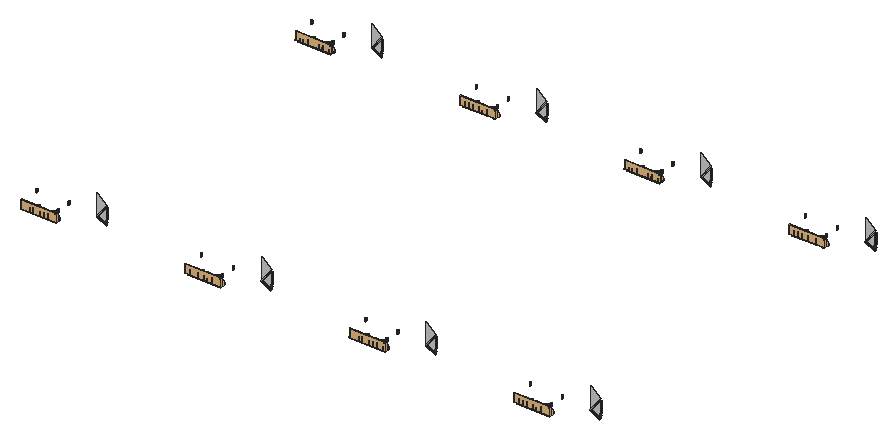
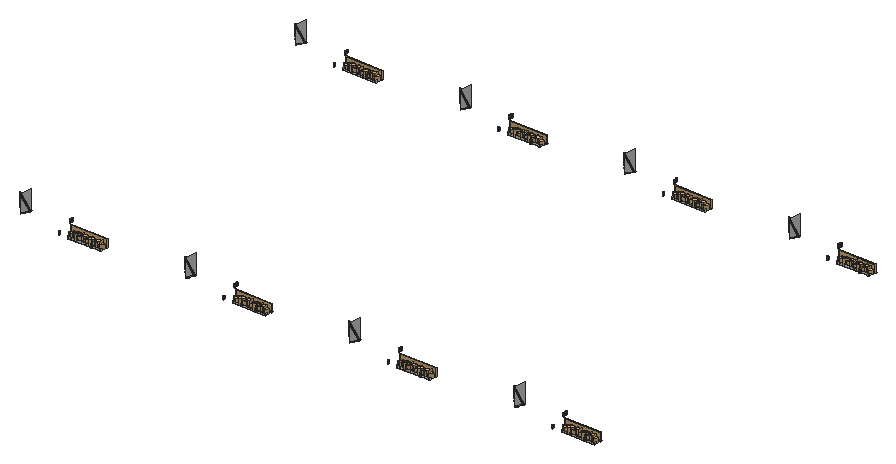
# SketchUp Ruby script. Lengths in inches.
U = 1.inch
M = Sketchup.active_model
def pt(a) = Geom::Point3d.new(a.map { |v| v * U })
def face(e, loops, mat)
  f = e.add_face(loops[0].map { |a| pt(a) })
  loops[1..].each { |l| e.add_face(l.map { |a| pt(a) }).erase! }
  f.material = f.back_material = mat if mat
  f
end
# faces: each face lists its corners as indices into pts; further lists are holes
def faces(e, pts, list, mat = nil) = list.each { |f| face(e, (f[0].is_a?(Array) ? f : [f]).map { |l| l.map { |i| pts[i] } }, mat) }
# xy, xz, yz: faces in a plane at the given z, y or x. An outline is a flat list of corners, or four numbers for a rectangle; further outlines are holes
def ring(l) = l.size == 4 ? [[l[0], l[1]], [l[2], l[1]], [l[2], l[3]], [l[0], l[3]]] : l.each_slice(2).to_a
def flat(e, list, mat, &to3) = list.each { |f| face(e, (f[0].is_a?(Array) ? f : [f]).map { |l| ring(l).map { |u, v| to3.(u, v) } }, mat) }
def xy(e, z, list, mat = nil) = flat(e, list, mat) { |x, y| [x, y, z] }
def xz(e, y, list, mat = nil) = flat(e, list, mat) { |x, z| [x, y, z] }
def yz(e, x, list, mat = nil) = flat(e, list, mat) { |y, z| [x, y, z] }
def lines(e, pts, list) = list.each { |a, b| e.add_line(pt(pts[a]), pt(pts[b])) }
# prism: a flat outline (further loops are holes) pulled along v
def prism(e, loops, v, mat = nil)
  f = face(e, loops, mat); d = Geom::Vector3d.new(v.map { |x| x * U })
  f.pushpull(f.normal.samedirection?(d) ? d.length : -d.length)
end
def box(e, o, s, mat = nil) = prism(e, [[o, [o[0] + s[0], o[1], o[2]], [o[0] + s[0], o[1] + s[1], o[2]], [o[0], o[1] + s[1], o[2]]]], [0, 0, s[2]], mat)
def at(x, y, z, deg = 0) = Geom::Transformation.translation(pt([x, y, z])) * Geom::Transformation.rotation(ORIGIN, Z_AXIS, deg.degrees)
def axes(o, x, y, z) = Geom::Transformation.new([*x, 0, *y, 0, *z, 0, *pt(o).to_a, 1])
def part(name) = M.definitions.add(name)
# library, detail: a bought-in or finely detailed component or shape, given as its bounding box
def library(name, o, s) = part(name).tap { |d| box(d.entities, o, s) }
def detail(e, o, s) = box(e.add_group.entities, o, s)
def put(e, d, t, mat = nil) = e.add_instance(d, t).tap { |i| i.material = mat if mat }
def group(e, t, mat = nil) = e.add_group.tap { |g| g.transformation = t; g.material = mat if mat }.entities
root = M.entities
M.materials.add("Material__1").color = [95, 70, 46]
M.materials.add("[Carrera Marble]").color = [207, 207, 207]
M.materials.add("[Field Square Tile]").color = [211, 167, 108]
M.materials.add("[Granite Dark Gray]").color = [38, 37, 37]
M.materials.add("[Granite Tile]1").color = [68, 65, 63]
c1 = library("Areca palm plant",[0,0,0],[49.1,36.6,54.46])
c2 = library("Group\#74",[-84.69,-90.07,-0.36],[176.51,175.13,171.4])
c3 = library("Group38\#2",[14.01,28.44,-23.43],[18.58,18.32,38.89])
c4 = library("Group\#130",[-7.34,-1.2,0],[38.67,35.81,49.04])
c5 = library("Group20\#1",[-20.81,-17.08,3.79],[39.86,39.43,37.51])
c6 = part("Group\#3")
xy(c6.entities,0,[[0,0,6,234.8],[30,0,36,234.8]])
xy(c6.entities,3,[[6,0,30,234.8]])
xy(c6.entities,7,[[6,5,30,229.8]],"Material__1")
xy(c6.entities,15,[[[0,0,36,234.8],[6,5,30,229.8]]])
xz(c6.entities,0,[[0,0,6,0,6,3,30,3,30,0,36,0,36,15,0,15]])
xz(c6.entities,5,[[6,7,30,15]])
xz(c6.entities,229.8,[[6,7,30,15]])
xz(c6.entities,234.8,[[0,0,0,15,36,15,36,0,30,0,30,3,6,3,6,0]])
yz(c6.entities,0,[[0,0,234.8,15]])
yz(c6.entities,6,[[0,0,234.8,3],[5,7,229.8,15]])
yz(c6.entities,30,[[0,0,234.8,3],[5,7,229.8,15]])
yz(c6.entities,36,[[0,0,234.8,15]])
c7 = part("Group\#5")
put(c7.entities,c1,axes([-6.2,158.41,6.08],[0.45017,-0.56191,0],[0.66137,0.52986,0],[0,0,0.72]))
put(c7.entities,c1,axes([-6.2,56.6,6.08],[0.45017,-0.56191,0],[0.66137,0.52986,0],[0,0,0.72]))
put(c7.entities,c2,axes([17.19,15.79,6.07],[-0.08133,-0.14087,0],[0.14087,-0.08133,0],[0,0,0.1725]))
put(c7.entities,c2,axes([14.93,173.12,6.05],[-0.04961,-0.08593,0],[0.08593,-0.04961,0],[0,0,0.10522]))
put(c7.entities,c2,axes([17.19,223.04,6.07],[-0.08133,-0.14087,0],[0.14087,-0.08133,0],[0,0,0.1725]))
put(c7.entities,c3,axes([-4.1,-1.15,28.17],[0.8848,0,0],[0,0.94674,0],[0,0,0.85826]))
put(c7.entities,c2,axes([14.93,193.18,6.05],[-0.04961,-0.08593,0],[0.08593,-0.04961,0],[0,0,0.10522]))
put(c7.entities,c2,axes([14.93,91.37,6.05],[-0.04961,-0.08593,0],[0.08593,-0.04961,0],[0,0,0.10522]))
put(c7.entities,c4,axes([24.9375,191.72,8],[0,0.79,0],[-0.79,0,0],[0,0,0.79]))
put(c7.entities,c5,axes([18.97,181.79,4.77],[0,0.85,0],[-0.85,0,0],[0,0,0.85]))
put(c7.entities,c2,axes([14.93,145.87,6.05],[-0.04961,-0.08593,0],[0.08593,-0.04961,0],[0,0,0.10522]))
put(c7.entities,c5,axes([18.97,79.98,4.77],[0,0.85,0],[-0.85,0,0],[0,0,0.85]))
put(c7.entities,c2,axes([14.93,71.3,6.05],[-0.04961,-0.08593,0],[0.08593,-0.04961,0],[0,0,0.10522]))
put(c7.entities,c4,axes([24.9375,89.91,8],[0,0.79,0],[-0.79,0,0],[0,0,0.79]))
put(c7.entities,c2,axes([14.93,44.05,6.05],[-0.04961,-0.08593,0],[0.08593,-0.04961,0],[0,0,0.10522]))
put(c7.entities,c2,axes([17.19,121.23,6.07],[-0.08133,-0.14087,0],[0.14087,-0.08133,0],[0,0,0.1725]))
put(c7.entities,c6,at(0,0,0))
put(c7.entities,c3,axes([-4.1,100.66,28.17],[0.8848,0,0],[0,0.94674,0],[0,0,0.85826]))
c8 = library("Glass Railing",[0,0,0],[139.5,4.76,42])
c9 = part("Group\#7")
xy(c9.entities,0,[[6,0,4.45,0.2,3,0.8,1.76,1.76,0.8,3,0.2,4.45,0,6,0.2,7.55,0.8,9,1.76,10.24,3,11.2,4.45,11.8,6,12,7.55,11.8,9,11.2,10.24,10.24,11.2,9,11.8,7.55,12,6,11.8,4.45,11.2,3,10.24,1.76,9,0.8,7.55,0.2]])
xy(c9.entities,37,[[6,0,7.55,0.2,9,0.8,10.24,1.76,11.2,3,11.8,4.45,12,6,11.8,7.55,11.2,9,10.24,10.24,9,11.2,7.55,11.8,6,12,4.45,11.8,3,11.2,1.76,10.24,0.8,9,0.2,7.55,0,6,0.2,4.45,0.8,3,1.76,1.76,3,0.8,4.45,0.2]],"[Granite Tile]1")
p = [[4.45,0.2,0],[6,0,0],[6,0,37],[4.45,0.2,37],[7.55,0.2,0],[7.55,0.2,37],
  [3,0.8,0],[3,0.8,37],[9,0.8,0],[9,0.8,37],[1.76,1.76,0],[1.76,1.76,37],
  [10.24,1.76,0],[10.24,1.76,37],[0.8,3,0],[0.8,3,37],[11.2,3,0],[11.2,3,37],
  [0.2,4.45,0],[0.2,4.45,37],[11.8,4.45,0],[11.8,4.45,37],[0,6,0],[0,6,37],
  [12,6,0],[12,6,37],[0.2,7.55,0],[0.2,7.55,37],[11.8,7.55,0],[11.8,7.55,37],
  [0.8,9,0],[0.8,9,37],[11.2,9,0],[11.2,9,37],[1.76,10.24,0],[1.76,10.24,37],
  [10.24,10.24,0],[10.24,10.24,37],[3,11.2,0],[3,11.2,37],[9,11.2,0],[9,11.2,37],
  [4.45,11.8,0],[4.45,11.8,37],[7.55,11.8,0],[7.55,11.8,37],[6,12,0],[6,12,37]]
faces(c9.entities,p,[[0,1,2,3],[1,4,5,2],[6,0,3,7],[4,8,9,5],[10,6,7,11],[8,12,13,9],[14,10,11,15],[12,16,17,13],
  [18,14,15,19],[16,20,21,17],[22,18,19,23],[20,24,25,21],[26,22,23,27],[24,28,29,25],[30,26,27,31],[28,32,33,29],
  [34,30,31,35],[32,36,37,33],[38,34,35,39],[36,40,41,37],[42,38,39,43],[40,44,45,41],[46,42,43,47],[44,46,47,45]],"[Granite Tile]1")
xy(root,147.6875,[[232.96,463.25,427.1,468.31],[1111.71,463.25,1305.85,468.31],[1990.46,463.25,2184.6,468.31],[2869.21,463.25,3063.35,468.31],[232.96,2298.875,427.1,2303.93],
  [1111.71,2298.875,1305.85,2303.93],[1990.46,2298.875,2184.6,2303.93],[2869.21,2298.875,3063.35,2303.93]])
xy(root,210.79,[[659.68,501.4,665.11,508.33],[1538.43,501.4,1543.86,508.33],[2417.18,501.4,2422.61,508.33],[3295.93,501.4,3301.36,508.33],[659.68,2337.02,665.11,2343.96],
  [1538.43,2337.02,1543.86,2343.96],[2417.18,2337.02,2422.61,2343.96],[3295.93,2337.02,3301.36,2343.96]],"[Granite Dark Gray]")
xy(root,223.24,[[659.68,501.4,665.11,508.33],[1538.43,501.4,1543.86,508.33],[2417.18,501.4,2422.61,508.33],[3295.93,501.4,3301.36,508.33],[659.68,2337.02,665.11,2343.96],
  [1538.43,2337.02,1543.86,2343.96],[2417.18,2337.02,2422.61,2343.96],[3295.93,2337.02,3301.36,2343.96]],"[Granite Dark Gray]")
xz(root,501.4,[[659.68,210.79,665.11,223.24],[1538.43,210.79,1543.86,223.24],[2417.18,210.79,2422.61,223.24],[3295.93,210.79,3301.36,223.24]],"[Granite Tile]1")
xz(root,508.33,[[659.68,223.24,665.11,282.18],[1538.43,223.24,1543.86,282.18],[2417.18,223.24,2422.61,282.18],[3295.93,223.24,3301.36,282.18]],"[Granite Dark Gray]")
xz(root,513.52,[[653.06,188.27,653.06,192.89,607.75,217.02,653.06,275.14,653.06,284.38,599.51,215.75],[1531.81,188.27,1531.81,192.89,1486.5,217.02,1531.81,275.14,1531.81,284.38,1478.26,215.75],[2410.56,188.27,2410.56,192.89,2365.25,217.02,2410.56,275.14,2410.56,284.38,2357.01,215.75],[3289.31,188.27,3289.31,192.89,3244,217.02,3289.31,275.14,3289.31,284.38,3235.76,215.75]],"[Field Square Tile]")
xz(root,518.65,[[653.06,192.89,653.06,275.14,607.75,217.02],[1531.81,192.89,1531.81,275.14,1486.5,217.02],[2410.56,192.89,2410.56,275.14,2365.25,217.02],[3289.31,192.89,3289.31,275.14,3244,217.02],[599.51,215.75,653.06,284.38,599.51,327.51],
  [1478.26,215.75,1531.81,284.38,1478.26,327.51],[2357.01,215.75,2410.56,284.38,2357.01,327.51],[3235.76,215.75,3289.31,284.38,3235.76,327.51]],"[Carrera Marble]")
xz(root,2337.02,[[659.68,210.79,665.11,223.24],[1538.43,210.79,1543.86,223.24],[2417.18,210.79,2422.61,223.24],[3295.93,210.79,3301.36,223.24]],"[Granite Tile]1")
xz(root,2343.96,[[659.68,223.24,665.11,282.18],[1538.43,223.24,1543.86,282.18],[2417.18,223.24,2422.61,282.18],[3295.93,223.24,3301.36,282.18]],"[Granite Dark Gray]")
xz(root,2349.15,[[653.06,188.27,653.06,192.89,607.75,217.02,653.06,275.14,653.06,284.38,599.51,215.75],[1531.81,188.27,1531.81,192.89,1486.5,217.02,1531.81,275.14,1531.81,284.38,1478.26,215.75],[2410.56,188.27,2410.56,192.89,2365.25,217.02,2410.56,275.14,2410.56,284.38,2357.01,215.75],[3289.31,188.27,3289.31,192.89,3244,217.02,3289.31,275.14,3289.31,284.38,3235.76,215.75]],"[Field Square Tile]")
xz(root,2354.27,[[653.06,192.89,653.06,275.14,607.75,217.02],[1531.81,192.89,1531.81,275.14,1486.5,217.02],[2410.56,192.89,2410.56,275.14,2365.25,217.02],[3289.31,192.89,3289.31,275.14,3244,217.02],[599.51,215.75,653.06,284.38,599.51,327.51],
  [1478.26,215.75,1531.81,284.38,1478.26,327.51],[2357.01,215.75,2410.56,284.38,2357.01,327.51],[3235.76,215.75,3289.31,284.38,3235.76,327.51]],"[Carrera Marble]")
p = [[599.51,518.65,215.75],[653.06,518.65,188.27],[653.06,513.52,188.27],[599.51,513.52,215.75],[1478.26,518.65,215.75],[1531.81,518.65,188.27],
  [1531.81,513.52,188.27],[1478.26,513.52,215.75],[2357.01,518.65,215.75],[2410.56,518.65,188.27],[2410.56,513.52,188.27],[2357.01,513.52,215.75],
  [3235.76,518.65,215.75],[3289.31,518.65,188.27],[3289.31,513.52,188.27],[3235.76,513.52,215.75],[599.51,2354.27,215.75],[653.06,2354.27,188.27],
  [653.06,2349.15,188.27],[599.51,2349.15,215.75],[1478.26,2354.27,215.75],[1531.81,2354.27,188.27],[1531.81,2349.15,188.27],[1478.26,2349.15,215.75],
  [2357.01,2354.27,215.75],[2410.56,2354.27,188.27],[2410.56,2349.15,188.27],[2357.01,2349.15,215.75],[3235.76,2354.27,215.75],[3289.31,2354.27,188.27],
  [3289.31,2349.15,188.27],[3235.76,2349.15,215.75],[653.06,518.65,192.89],[607.75,518.65,217.02],[607.75,513.52,217.02],[653.06,513.52,192.89],
  [1531.81,518.65,192.89],[1486.5,518.65,217.02],[1486.5,513.52,217.02],[1531.81,513.52,192.89],[2410.56,518.65,192.89],[2365.25,518.65,217.02],
  [2365.25,513.52,217.02],[2410.56,513.52,192.89],[3289.31,518.65,192.89],[3244,518.65,217.02],[3244,513.52,217.02],[3289.31,513.52,192.89],
  [653.06,2354.27,192.89],[607.75,2354.27,217.02],[607.75,2349.15,217.02],[653.06,2349.15,192.89],[1531.81,2354.27,192.89],[1486.5,2354.27,217.02],
  [1486.5,2349.15,217.02],[1531.81,2349.15,192.89],[2410.56,2354.27,192.89],[2365.25,2354.27,217.02],[2365.25,2349.15,217.02],[2410.56,2349.15,192.89],
  [3289.31,2354.27,192.89],[3244,2354.27,217.02],[3244,2349.15,217.02],[3289.31,2349.15,192.89],[653.06,518.65,284.38],[653.06,513.52,284.38],
  [1531.81,518.65,284.38],[1531.81,513.52,284.38],[2410.56,518.65,284.38],[2410.56,513.52,284.38],[3289.31,518.65,284.38],[3289.31,513.52,284.38],
  [653.06,2354.27,284.38],[653.06,2349.15,284.38],[1531.81,2354.27,284.38],[1531.81,2349.15,284.38],[2410.56,2354.27,284.38],[2410.56,2349.15,284.38],
  [3289.31,2354.27,284.38],[3289.31,2349.15,284.38],[653.06,518.65,275.14],[653.06,513.52,275.14],[1531.81,518.65,275.14],[1531.81,513.52,275.14],
  [2410.56,518.65,275.14],[2410.56,513.52,275.14],[3289.31,518.65,275.14],[3289.31,513.52,275.14],[653.06,2354.27,275.14],[653.06,2349.15,275.14],
  [1531.81,2354.27,275.14],[1531.81,2349.15,275.14],[2410.56,2354.27,275.14],[2410.56,2349.15,275.14],[3289.31,2354.27,275.14],[3289.31,2349.15,275.14]]
faces(root,p,[[0,1,2,3],[4,5,6,7],[8,9,10,11],[12,13,14,15],[16,17,18,19],[20,21,22,23],[24,25,26,27],[28,29,30,31],
  [32,33,34,35],[36,37,38,39],[40,41,42,43],[44,45,46,47],[48,49,50,51],[52,53,54,55],[56,57,58,59],[60,61,62,63],
  [64,0,3,65],[66,4,7,67],[68,8,11,69],[70,12,15,71],[72,16,19,73],[74,20,23,75],[76,24,27,77],[78,28,31,79],
  [33,80,81,34],[37,82,83,38],[41,84,85,42],[45,86,87,46],[49,88,89,50],[53,90,91,54],[57,92,93,58],[61,94,95,62]])
put(root,c7,axes([2177.86,467.88,140.63],[0,0.7469,0],[-0.7469,0,0],[0,0,0.7469]))
put(root,c7,axes([3056.61,467.88,140.63],[0,0.7469,0],[-0.7469,0,0],[0,0,0.7469]))
put(root,c7,axes([1299.11,467.88,140.63],[0,0.7469,0],[-0.7469,0,0],[0,0,0.7469]))
put(root,c7,axes([420.36,467.88,140.63],[0,0.7469,0],[-0.7469,0,0],[0,0,0.7469]))
put(root,c7,axes([3056.61,2303.5,140.63],[0,0.7469,0],[-0.7469,0,0],[0,0,0.7469]))
put(root,c7,axes([2177.86,2303.5,140.63],[0,0.7469,0],[-0.7469,0,0],[0,0,0.7469]))
put(root,c7,axes([420.36,2303.5,140.63],[0,0.7469,0],[-0.7469,0,0],[0,0,0.7469]))
put(root,c7,axes([1299.11,2303.5,140.63],[0,0.7469,0],[-0.7469,0,0],[0,0,0.7469]))
put(root,c8,axes([1992.04,463.25,147.6875],[1.38033,0,0],[0,1,0],[0,0,1]))
put(root,c8,axes([2870.79,463.25,147.6875],[1.38033,0,0],[0,1,0],[0,0,1]))
put(root,c8,axes([234.54,463.25,147.6875],[1.38033,0,0],[0,1,0],[0,0,1]))
put(root,c8,axes([1113.29,463.25,147.6875],[1.38033,0,0],[0,1,0],[0,0,1]))
put(root,c8,axes([1992.04,2298.875,147.6875],[1.38033,0,0],[0,1,0],[0,0,1]))
put(root,c8,axes([1113.29,2298.875,147.6875],[1.38033,0,0],[0,1,0],[0,0,1]))
put(root,c8,axes([234.54,2298.875,147.6875],[1.38033,0,0],[0,1,0],[0,0,1]))
put(root,c8,axes([2870.79,2298.875,147.6875],[1.38033,0,0],[0,1,0],[0,0,1]))
put(root,c9,axes([2171.3,556.01,187.92],[0.42,0,0],[0,0.42,0],[0,0,0.42]))
put(root,c9,axes([2000.11,556.01,187.92],[0.42,0,0],[0,0.42,0],[0,0,0.42]))
put(root,c9,axes([3050.05,556.01,187.92],[0.42,0,0],[0,0.42,0],[0,0,0.42]))
put(root,c9,axes([2878.86,556.01,187.92],[0.42,0,0],[0,0.42,0],[0,0,0.42]))
put(root,c9,axes([413.8,556.01,187.92],[0.42,0,0],[0,0.42,0],[0,0,0.42]))
put(root,c9,axes([1292.55,556.01,187.92],[0.42,0,0],[0,0.42,0],[0,0,0.42]))
put(root,c9,axes([1121.36,556.01,187.92],[0.42,0,0],[0,0.42,0],[0,0,0.42]))
put(root,c9,axes([242.61,556.01,187.92],[0.42,0,0],[0,0.42,0],[0,0,0.42]))
put(root,c9,axes([2171.3,2391.64,187.92],[0.42,0,0],[0,0.42,0],[0,0,0.42]))
put(root,c9,axes([3050.05,2391.64,187.92],[0.42,0,0],[0,0.42,0],[0,0,0.42]))
put(root,c9,axes([2878.86,2391.64,187.92],[0.42,0,0],[0,0.42,0],[0,0,0.42]))
put(root,c9,axes([2000.11,2391.64,187.92],[0.42,0,0],[0,0.42,0],[0,0,0.42]))
put(root,c9,axes([1121.36,2391.64,187.92],[0.42,0,0],[0,0.42,0],[0,0,0.42]))
put(root,c9,axes([413.8,2391.64,187.92],[0.42,0,0],[0,0.42,0],[0,0,0.42]))
put(root,c9,axes([1292.55,2391.64,187.92],[0.42,0,0],[0,0.42,0],[0,0,0.42]))
put(root,c9,axes([242.61,2391.64,187.92],[0.42,0,0],[0,0.42,0],[0,0,0.42]))
put(root,c9,axes([2188.83,458.5,197.42],[0.42,0,0],[0,0.42,0],[0,0,0.42]))
put(root,c9,axes([2188.92,460.37,197.42],[0.42,0,0],[0,0.42,0],[0,0,0.42]))
put(root,c9,axes([2189.4375,446.5625,197.42],[0.42,0,0],[0,0.42,0],[0,0,0.42]))
put(root,c9,axes([3067.67,460.37,197.42],[0.42,0,0],[0,0.42,0],[0,0,0.42]))
put(root,c9,axes([3067.58,458.5,197.42],[0.42,0,0],[0,0.42,0],[0,0,0.42]))
put(root,c9,axes([3068.1875,446.5625,197.42],[0.42,0,0],[0,0.42,0],[0,0,0.42]))
put(root,c9,axes([431.42,460.37,197.42],[0.42,0,0],[0,0.42,0],[0,0,0.42]))
put(root,c9,axes([431.33,458.5,197.42],[0.42,0,0],[0,0.42,0],[0,0,0.42]))
put(root,c9,axes([1310.17,460.37,197.42],[0.42,0,0],[0,0.42,0],[0,0,0.42]))
put(root,c9,axes([1310.6875,446.5625,197.42],[0.42,0,0],[0,0.42,0],[0,0,0.42]))
put(root,c9,axes([1310.08,458.5,197.42],[0.42,0,0],[0,0.42,0],[0,0,0.42]))
put(root,c9,axes([431.9375,446.5625,197.42],[0.42,0,0],[0,0.42,0],[0,0,0.42]))
put(root,c9,axes([2188.92,2295.99,197.42],[0.42,0,0],[0,0.42,0],[0,0,0.42]))
put(root,c9,axes([2188.83,2294.125,197.42],[0.42,0,0],[0,0.42,0],[0,0,0.42]))
put(root,c9,axes([3067.67,2295.99,197.42],[0.42,0,0],[0,0.42,0],[0,0,0.42]))
put(root,c9,axes([3068.1875,2282.1875,197.42],[0.42,0,0],[0,0.42,0],[0,0,0.42]))
put(root,c9,axes([3067.58,2294.125,197.42],[0.42,0,0],[0,0.42,0],[0,0,0.42]))
put(root,c9,axes([2189.4375,2282.1875,197.42],[0.42,0,0],[0,0.42,0],[0,0,0.42]))
put(root,c9,axes([431.33,2294.125,197.42],[0.42,0,0],[0,0.42,0],[0,0,0.42]))
put(root,c9,axes([431.42,2295.99,197.42],[0.42,0,0],[0,0.42,0],[0,0,0.42]))
put(root,c9,axes([431.9375,2282.1875,197.42],[0.42,0,0],[0,0.42,0],[0,0,0.42]))
put(root,c9,axes([1310.17,2295.99,197.42],[0.42,0,0],[0,0.42,0],[0,0,0.42]))
put(root,c9,axes([1310.08,2294.125,197.42],[0.42,0,0],[0,0.42,0],[0,0,0.42]))
put(root,c9,axes([1310.6875,2282.1875,197.42],[0.42,0,0],[0,0.42,0],[0,0,0.42]))
